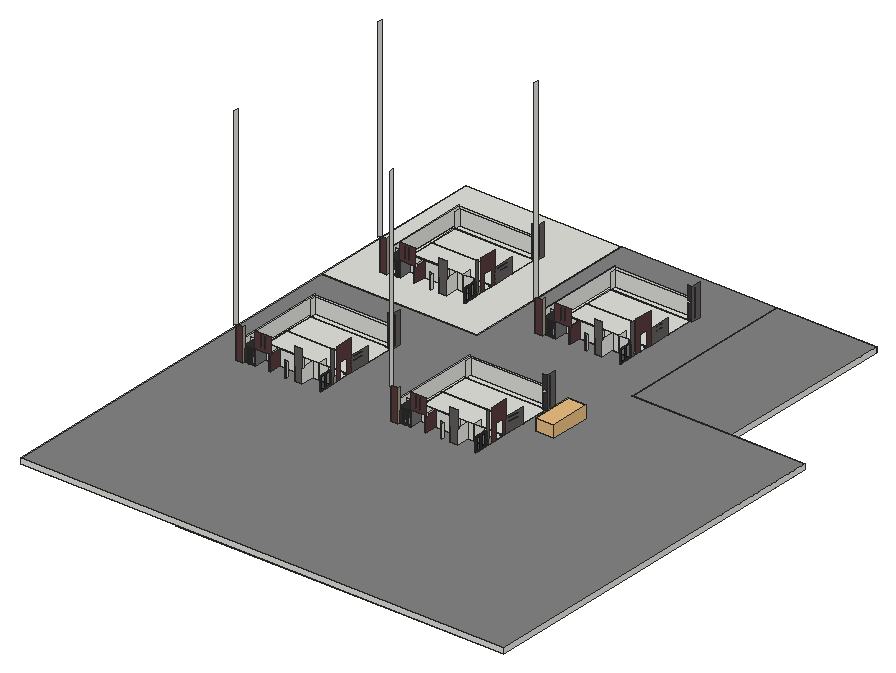
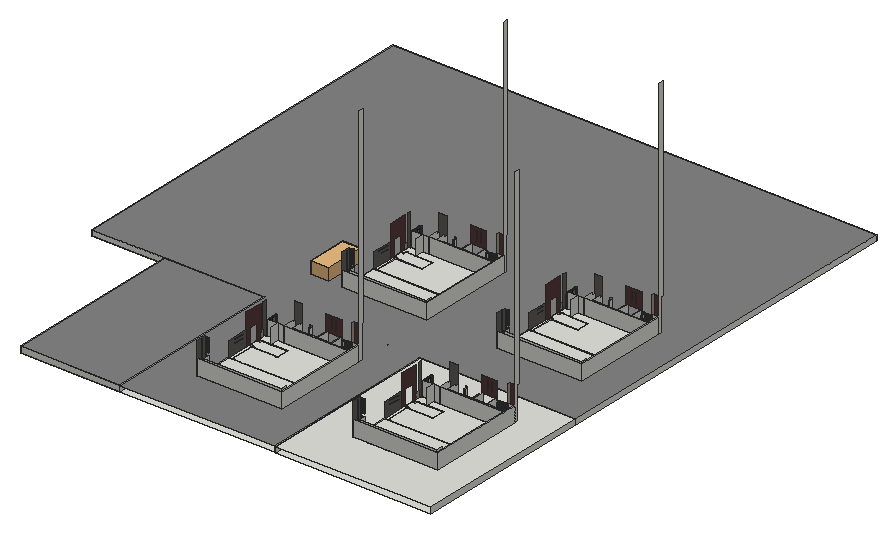
# SketchUp Ruby script. Lengths in inches.
U = 1.inch
M = Sketchup.active_model
def pt(a) = Geom::Point3d.new(a.map { |v| v * U })
def face(e, loops, mat)
  f = e.add_face(loops[0].map { |a| pt(a) })
  loops[1..].each { |l| e.add_face(l.map { |a| pt(a) }).erase! }
  f.material = f.back_material = mat if mat
  f
end
# faces: each face lists its corners as indices into pts; further lists are holes
def faces(e, pts, list, mat = nil) = list.each { |f| face(e, (f[0].is_a?(Array) ? f : [f]).map { |l| l.map { |i| pts[i] } }, mat) }
# xy, xz, yz: faces in a plane at the given z, y or x. An outline is a flat list of corners, or four numbers for a rectangle; further outlines are holes
def ring(l) = l.size == 4 ? [[l[0], l[1]], [l[2], l[1]], [l[2], l[3]], [l[0], l[3]]] : l.each_slice(2).to_a
def flat(e, list, mat, &to3) = list.each { |f| face(e, (f[0].is_a?(Array) ? f : [f]).map { |l| ring(l).map { |u, v| to3.(u, v) } }, mat) }
def xy(e, z, list, mat = nil) = flat(e, list, mat) { |x, y| [x, y, z] }
def xz(e, y, list, mat = nil) = flat(e, list, mat) { |x, z| [x, y, z] }
def yz(e, x, list, mat = nil) = flat(e, list, mat) { |y, z| [x, y, z] }
def lines(e, pts, list) = list.each { |a, b| e.add_line(pt(pts[a]), pt(pts[b])) }
# prism: a flat outline (further loops are holes) pulled along v
def prism(e, loops, v, mat = nil)
  f = face(e, loops, mat); d = Geom::Vector3d.new(v.map { |x| x * U })
  f.pushpull(f.normal.samedirection?(d) ? d.length : -d.length)
end
def box(e, o, s, mat = nil) = prism(e, [[o, [o[0] + s[0], o[1], o[2]], [o[0] + s[0], o[1] + s[1], o[2]], [o[0], o[1] + s[1], o[2]]]], [0, 0, s[2]], mat)
def at(x, y, z, deg = 0) = Geom::Transformation.translation(pt([x, y, z])) * Geom::Transformation.rotation(ORIGIN, Z_AXIS, deg.degrees)
def axes(o, x, y, z) = Geom::Transformation.new([*x, 0, *y, 0, *z, 0, *pt(o).to_a, 1])
def part(name) = M.definitions.add(name)
# library, detail: a bought-in or finely detailed component or shape, given as its bounding box
def library(name, o, s) = part(name).tap { |d| box(d.entities, o, s) }
def detail(e, o, s) = box(e.add_group.entities, o, s)
def put(e, d, t, mat = nil) = e.add_instance(d, t).tap { |i| i.material = mat if mat }
def group(e, t, mat = nil) = e.add_group.tap { |g| g.transformation = t; g.material = mat if mat }.entities
root = M.entities
M.materials.add("Glass_Tinted_Gray").color = [0, 0, 0]
M.materials["Glass_Tinted_Gray"].alpha = 0.125
M.materials.add("Wine2").color = [0, 0, 0]
M.materials["Wine2"].alpha = 0
M.materials.add("[0130_Gainsboro]").color = [39, 45, 50]
M.materials.add("[0135_DarkGray]").color = [81, 81, 81]
M.materials.add("[Color M05]").color = [114, 114, 114]
M.materials.add("[Color M07]").color = [58, 58, 58]
M.materials.add("[Concrete Tile]").color = [165, 155, 133]
M.materials.add("[Granite Brown]").color = [89, 59, 61]
M.materials.add("[Mirror 02]").color = [229, 229, 229]
M.materials.add("[Stone Marble]").color = [99, 95, 94]
M.materials.add("[Terrazzo Light Blue]").color = [196, 214, 227]
M.materials.add("[Tile Grey]").color = [132, 132, 132]
c1 = part("PENTEK_RP Fineline 50S_Sliding_DoorCase_E1")
box(c1.entities,[0,0,0],[1.51,3.66,99.27],"[0135_DarkGray]")
c2 = part("PENTEK_RP Fineline 50S_SlidingDooe_Case_E2")
box(c2.entities,[0,0,0],[96.25,3.66,1.51],"[0135_DarkGray]")
c3 = part("pentek_RP Fineline 50S_SlidingDoor_Case")
put(c3.entities,c1,at(97.76,0,0))
put(c3.entities,c2,at(1.51,0,0))
put(c3.entities,c1,at(0,0,0))
put(c3.entities,c2,at(1.51,0,97.76))
c4 = part("PENTEK_RP Fineline 50S_SlidingDoor_GlazingBead_2")
box(c4.entities,[0,0,0],[0.56,0.59,94.39],"[0135_DarkGray]")
c5 = part("PENTEK_RP Fineline 50S_SlidingDoor_Glass")
box(c5.entities,[0,0,0],[46.58,0.16,94.39],"Glass_Tinted_Gray")
c6 = part("PENTEK_RP Fineline 50S_SlidingDoor_GlazingBead")
box(c6.entities,[0,0,0],[45.47,0.59,0.56],"[0135_DarkGray]")
c7 = part("PENTEK_RP Fineline 50S_SlidingDoor_Leaf_E1")
xy(c7.entities,0,[[0,0,0.93,1.97],[0.93,1.57,1.49,1.97]],"[0135_DarkGray]")
xy(c7.entities,96.25,[[0,0,0.93,0,0.93,1.57,1.49,1.57,1.49,1.97,0,1.97]],"[0135_DarkGray]")
xz(c7.entities,0,[[0,0,0.93,96.25]],"[0135_DarkGray]")
xz(c7.entities,1.57,[[0.93,0,1.49,95.32],[0.93,95.32,1.49,96.25]],"[0135_DarkGray]")
xz(c7.entities,1.97,[[0,0,1.49,96.25]],"[0135_DarkGray]")
yz(c7.entities,0,[[0,0,1.97,96.25]],"[0135_DarkGray]")
yz(c7.entities,0.93,[[0,0,1.57,0.93],[0,0.93,1.57,95.32],[0,95.32,1.57,96.25]],"[0135_DarkGray]")
yz(c7.entities,1.49,[[1.57,0,1.97,95.32],[1.57,95.32,1.97,96.25]],"[0135_DarkGray]")
c8 = part("PENTEK_RP Fineline 50S_SlidingDoor_Leaf_E2")
xy(c8.entities,0,[[0,0,0,1.57,0.56,1.57,0.56,1.97,46.02,1.97,46.02,1.57,46.58,1.57,46.58,0]],"[0135_DarkGray]")
xy(c8.entities,0.93,[[0,0,46.58,1.57]],"[0135_DarkGray]")
xy(c8.entities,1.49,[[0.56,1.57,46.02,1.97]],"[0135_DarkGray]")
xz(c8.entities,0,[[0,0,46.58,0.93]],"[0135_DarkGray]")
xz(c8.entities,1.57,[[0,0,0.56,0.93],[46.02,0,46.58,0.93],[0.56,0.93,46.02,1.49]],"[0135_DarkGray]")
xz(c8.entities,1.97,[[0.56,0,46.02,1.49]],"[0135_DarkGray]")
yz(c8.entities,0,[[0,0,1.57,0.93]],"[0135_DarkGray]")
yz(c8.entities,0.56,[[1.57,0,1.97,0.93],[1.57,0.93,1.97,1.49]],"[0135_DarkGray]")
yz(c8.entities,46.02,[[1.57,0,1.97,0.93],[1.57,0.93,1.97,1.49]],"[0135_DarkGray]")
yz(c8.entities,46.58,[[0,0,1.57,0.93]],"[0135_DarkGray]")
c9 = part("PENTEK_RP Fineline S_SlidingDoor_Leaf1")
put(c9.entities,c4,at(0.93,0,0.93))
put(c9.entities,c4,at(46.96,0,0.93))
put(c9.entities,c5,at(1.49,1.42,0.93))
put(c9.entities,c6,at(1.49,0,0.93))
put(c9.entities,c5,at(1.49,0.59,0.93),"[Terrazzo Light Blue]")
put(c9.entities,c7,at(0,0,0))
put(c9.entities,c7,axes([48.44,0,0],[-1,0,0],[0,1,0],[0,0,1]))
put(c9.entities,c8,axes([0.93,0,96.25],[1,0,0],[0,1,0],[0,0,-1]))
put(c9.entities,c8,at(0.93,0,0))
put(c9.entities,c6,at(1.49,0,94.77))
c10 = part("PENTEK_RP Fineline 50S_SlidingDoor_Leaf2")
put(c10.entities,c5,at(1.49,1.42,0.93))
put(c10.entities,c6,at(1.49,0,94.77))
put(c10.entities,c4,at(46.96,0,0.93))
put(c10.entities,c5,at(1.49,0.59,0.93),"[Mirror 02]")
put(c10.entities,c4,at(0.93,0,0.93))
put(c10.entities,c7,at(0,0,0))
put(c10.entities,c7,axes([48.44,0,0],[-1,0,0],[0,1,0],[0,0,1]))
put(c10.entities,c6,at(1.49,0,0.93))
put(c10.entities,c8,axes([0.93,0,96.25],[1,0,0],[0,1,0],[0,0,-1]))
put(c10.entities,c8,at(0.93,0,0))
c11 = part("PENTEK - Slimmest Steel Sliding Door / Window\#1")
put(c11.entities,c3,at(0,-1.88,-0.09))
put(c11.entities,c9,at(1.51,-2.27,1.42))
put(c11.entities,c10,at(49.32,-0.3,1.42))
c12 = library("Group\#4",[0,0,0],[85.51,189.4,58.01])
c13 = part("2022 BMW i4")
put(c13.entities,c12,axes([0,0,0],[5,0,0],[0,5,0],[0,0,5]))
c14 = part("Framed glazing panel")
xy(c14.entities,0,[[0,-0.98,43.07,0],[0,0,43.07,1.4]],"[0130_Gainsboro]")
xy(c14.entities,0.3,[[0.3,-1.43,42.77,-0.98]],"[0130_Gainsboro]")
xy(c14.entities,2.95,[[2.95,-1.43,40.12,-0.63],[2.95,-0.63,40.12,0],[2.95,0,40.12,0.64],[2.95,0.64,40.12,1.4]],"[0130_Gainsboro]")
xy(c14.entities,3.54,[[3.54,-0.63,39.53,0],[3.54,0,39.53,0.64]],"[0130_Gainsboro]")
xy(c14.entities,111.8125,[[3.54,-0.63,39.53,0],[3.54,0,39.53,0.64]],"[0130_Gainsboro]")
xy(c14.entities,112.4,[[2.95,-1.43,40.12,-0.63],[2.95,-0.63,40.12,0],[2.95,0,40.12,0.64],[2.95,0.64,40.12,1.4]],"[0130_Gainsboro]")
xy(c14.entities,115.05,[[0.3,-1.43,42.77,-0.98]],"[0130_Gainsboro]")
xy(c14.entities,115.35,[[0,-0.98,43.07,0],[0,0,43.07,1.4]],"[0130_Gainsboro]")
xz(c14.entities,-1.43,[[[0.3,0.3,42.77,115.05],[2.95,2.95,40.12,112.4]]],"[0130_Gainsboro]")
xz(c14.entities,-0.98,[[[0,0,43.07,115.35],[0.3,0.3,42.77,115.05]]],"[0130_Gainsboro]")
xz(c14.entities,-0.63,[[[2.95,2.95,40.12,112.4],[3.54,3.54,39.53,111.8125]]],"[0130_Gainsboro]")
xz(c14.entities,0,[[3.54,3.54,39.53,111.8125]],"Wine2")
xz(c14.entities,0,[[[0,0,43.07,115.35],[2.95,2.95,40.12,112.4]],[[2.95,2.95,40.12,112.4],[3.54,3.54,39.53,111.8125]]],"[0130_Gainsboro]")
xz(c14.entities,0.64,[[[2.95,2.95,40.12,112.4],[3.54,3.54,39.53,111.8125]]],"[0130_Gainsboro]")
xz(c14.entities,1.4,[[[0,0,43.07,115.35],[2.95,2.95,40.12,112.4]]],"[0130_Gainsboro]")
yz(c14.entities,0,[[-0.98,0,0,115.35],[0,0,1.4,115.35]],"[0130_Gainsboro]")
yz(c14.entities,0.3,[[-1.43,0.3,-0.98,115.05]],"[0130_Gainsboro]")
yz(c14.entities,2.95,[[-1.43,2.95,-0.63,112.4],[-0.63,2.95,0,112.4],[0,2.95,0.64,112.4],[0.64,2.95,1.4,112.4]],"[0130_Gainsboro]")
yz(c14.entities,3.54,[[-0.63,3.54,0,111.8125],[0,3.54,0.64,111.8125]],"[0130_Gainsboro]")
yz(c14.entities,39.53,[[-0.63,3.54,0,111.8125],[0,3.54,0.64,111.8125]],"[0130_Gainsboro]")
yz(c14.entities,40.12,[[-1.43,2.95,-0.63,112.4],[-0.63,2.95,0,112.4],[0,2.95,0.64,112.4],[0.64,2.95,1.4,112.4]],"[0130_Gainsboro]")
yz(c14.entities,42.77,[[-1.43,0.3,-0.98,115.05]],"[0130_Gainsboro]")
yz(c14.entities,43.07,[[-0.98,0,0,115.35],[0,0,1.4,115.35]],"[0130_Gainsboro]")
c15 = part("Glazed panel assembly")
put(c15.entities,c14,axes([90.57,1.43,0],[1.05148,0,0],[0,1,0],[0,0,1]))
put(c15.entities,c14,axes([0,1.43,0],[1.05148,0,0],[0,1,0],[0,0,1]))
put(c15.entities,c14,axes([45.29,1.43,0],[1.05148,0,0],[0,1,0],[0,0,1]))
xy(root,-36.6875,[[0,0,1218.1875,2946.875],[1218.1875,0,1220.8125,2946.875],[1220.8125,0,3787.0625,2946.875],[0,2946.875,1218.1875,4361.5625],[1218.1875,2946.875,1220.8125,4361.5625],
  [1220.8125,2946.875,2436.375,4361.5625],[2439,2946.875,3218.5,4361.5625]])
xy(root,6,[[262.875,1778.3125,319.53,1799.9375],[1481.0625,1778.3125,1537.72,1799.9375],[262.875,1799.9375,262.875,2554.375,927.75,2554.375,927.75,2483.21,890.875,2483.21,890.875,2531.375,285.875,2531.375,285.875,1902.66,767.19,1902.66,767.19,1799.9375,709.87,1799.9375,709.87,1893.25,521.59,1893.25,521.59,1799.9375,511.23,1799.9375,511.23,1893.25,406.68,1893.25,406.68,1799.9375,399.88,1799.9375,399.88,1893.25,319.53,1893.25,319.53,1799.9375],[634.11,1799.9375,647.8,1814.92],[1481.0625,1799.9375,1481.0625,2554.375,2145.9375,2554.375,2145.9375,2483.21,2109.0625,2483.21,2109.0625,2531.375,1504.0625,2531.375,1504.0625,1902.66,1985.38,1902.66,1985.38,1799.9375,1928.05,1799.9375,1928.05,1893.25,1739.78,1893.25,1739.78,1799.9375,1729.42,1799.9375,1729.42,1893.25,1624.87,1893.25,1624.87,1799.9375,1618.07,1799.9375,1618.07,1893.25,1537.72,1893.25,1537.72,1799.9375],
  [1852.3,1799.9375,1865.99,1814.92],[285.875,1902.66,817,1902.66,817,1970.91,683.6875,1970.91,683.6875,2070.28,890.875,2070.28,890.875,2257.8125,285.875,2257.8125],[817,1902.66,817,1970.91,890.875,1970.91,890.875,1987.85,913.875,1987.85,913.875,1902.66],[1504.0625,1902.66,2035.1875,1902.66,2035.1875,1970.91,1901.875,1970.91,1901.875,2070.28,2109.0625,2070.28,2109.0625,2257.8125,1504.0625,2257.8125],[2035.1875,1902.66,2035.1875,1970.91,2109.0625,1970.91,2109.0625,1987.85,2132.0625,1987.85,2132.0625,1902.66],
  [683.6875,1970.91,683.6875,2070.28,890.875,2070.28,890.875,2059.15,913.875,2059.15,913.875,1987.85,890.875,1987.85,890.875,1970.91],[1901.875,1970.91,1901.875,2070.28,2109.0625,2070.28,2109.0625,2059.15,2132.0625,2059.15,2132.0625,1987.85,2109.0625,1987.85,2109.0625,1970.91],[890.875,2059.15,913.875,2257.8125],[2109.0625,2059.15,2132.0625,2257.8125],[285.875,2257.8125,285.875,2485.84,890.875,2485.84,890.875,2483.21,913.875,2483.21,913.875,2257.8125],
  [1504.0625,2257.8125,1504.0625,2485.84,2109.0625,2485.84,2109.0625,2483.21,2132.0625,2483.21,2132.0625,2257.8125],[285.875,2485.84,890.875,2531.375],[1504.0625,2485.84,2109.0625,2531.375],[0,2946.875,1218.1875,2946.875,1218.1875,4361.5625,262.875,4361.5625,262.875,3969.0625,927.75,3969.0625,927.75,3897.9,913.875,3897.9,913.875,3317.34,767.19,3317.34,767.19,3214.625,709.87,3214.625,709.87,3307.9375,634.11,3307.9375,634.11,3229.61,647.8,3229.61,647.8,3214.625,634.11,3214.625,634.11,3307.9375,521.59,3307.9375,521.59,3214.625,511.23,3214.625,511.23,3307.9375,406.68,3307.9375,406.68,3214.625,399.88,3214.625,399.88,3307.9375,319.53,3307.9375,319.53,3193,262.875,3193,262.875,4361.5625,0,4361.5625],[1218.1875,2946.875,1220.8125,4361.5625],
  [262.875,3193,319.53,3214.625],[1481.0625,3193,1537.72,3214.625],[262.875,3214.625,262.875,3969.0625,927.75,3969.0625,927.75,3897.9,890.875,3897.9,890.875,3946.0625,285.875,3946.0625,285.875,3317.34,767.19,3317.34,767.19,3214.625,709.87,3214.625,709.87,3307.9375,521.59,3307.9375,521.59,3214.625,511.23,3214.625,511.23,3307.9375,406.68,3307.9375,406.68,3214.625,399.88,3214.625,399.88,3307.9375,319.53,3307.9375,319.53,3214.625],[634.11,3214.625,647.8,3229.61],[1481.0625,3214.625,1481.0625,3969.0625,2145.9375,3969.0625,2145.9375,3897.9,2109.0625,3897.9,2109.0625,3946.0625,1504.0625,3946.0625,1504.0625,3317.34,1985.38,3317.34,1985.38,3214.625,1928.05,3214.625,1928.05,3307.9375,1739.78,3307.9375,1739.78,3214.625,1729.42,3214.625,1729.42,3307.9375,1624.87,3307.9375,1624.87,3214.625,1618.07,3214.625,1618.07,3307.9375,1537.72,3307.9375,1537.72,3214.625],
  [1852.3,3214.625,1865.99,3229.61],[285.875,3317.34,817,3317.34,817,3385.6,683.6875,3385.6,683.6875,3484.97,890.875,3484.97,890.875,3672.5,285.875,3672.5],[817,3317.34,817,3385.6,890.875,3385.6,890.875,3402.54,913.875,3402.54,913.875,3317.34],[1504.0625,3317.34,2035.1875,3317.34,2035.1875,3385.6,1901.875,3385.6,1901.875,3484.97,2109.0625,3484.97,2109.0625,3672.5,1504.0625,3672.5],[2035.1875,3317.34,2035.1875,3385.6,2109.0625,3385.6,2109.0625,3402.54,2132.0625,3402.54,2132.0625,3317.34],
  [683.6875,3385.6,683.6875,3484.97,890.875,3484.97,890.875,3473.84,913.875,3473.84,913.875,3402.54,890.875,3402.54,890.875,3385.6],[1901.875,3385.6,1901.875,3484.97,2109.0625,3484.97,2109.0625,3473.84,2132.0625,3473.84,2132.0625,3402.54,2109.0625,3402.54,2109.0625,3385.6],[890.875,3473.84,913.875,3672.5],[2109.0625,3473.84,2132.0625,3672.5],[285.875,3672.5,285.875,3900.52,890.875,3900.52,890.875,3897.9,913.875,3897.9,913.875,3672.5],
  [1504.0625,3672.5,1504.0625,3900.52,2109.0625,3900.52,2109.0625,3897.9,2132.0625,3897.9,2132.0625,3672.5],[285.875,3900.52,890.875,3946.0625],[1504.0625,3900.52,2109.0625,3946.0625]])
xy(root,6,[[0,0,3787.0625,0,3787.0625,2946.875,2436.375,2946.875,2436.375,4361.5625,1481.0625,4361.5625,1481.0625,3969.0625,2145.9375,3969.0625,2145.9375,3897.9,2132.0625,3897.9,2132.0625,3317.34,1985.38,3317.34,1985.38,3214.625,1928.05,3214.625,1928.05,3307.9375,1852.3,3307.9375,1852.3,3229.61,1865.99,3229.61,1865.99,3214.625,1852.3,3214.625,1852.3,3307.9375,1739.78,3307.9375,1739.78,3214.625,1729.42,3214.625,1729.42,3307.9375,1624.87,3307.9375,1624.87,3214.625,1618.07,3214.625,1618.07,3307.9375,1537.72,3307.9375,1537.72,3193,1481.0625,3193,1481.0625,4361.5625,1220.8125,4361.5625,1220.8125,2946.875,1481.0625,2946.875,1481.0625,2554.375,2145.9375,2554.375,2145.9375,2483.21,2132.0625,2483.21,2132.0625,1902.66,1985.38,1902.66,1985.38,1799.9375,1928.05,1799.9375,1928.05,1893.25,1852.3,1893.25,1852.3,1814.92,1865.99,1814.92,1865.99,1799.9375,1852.3,1799.9375,1852.3,1893.25,1739.78,1893.25,1739.78,1799.9375,1729.42,1799.9375,1729.42,1893.25,1624.87,1893.25,1624.87,1799.9375,1618.07,1799.9375,1618.07,1893.25,1537.72,1893.25,1537.72,1778.3125,1481.0625,1778.3125,1481.0625,2946.875,262.875,2946.875,262.875,2554.375,927.75,2554.375,927.75,2483.21,913.875,2483.21,913.875,1902.66,767.19,1902.66,767.19,1799.9375,709.87,1799.9375,709.87,1893.25,634.11,1893.25,634.11,1814.92,647.8,1814.92,647.8,1799.9375,634.11,1799.9375,634.11,1893.25,521.59,1893.25,521.59,1799.9375,511.23,1799.9375,511.23,1893.25,406.68,1893.25,406.68,1799.9375,399.88,1799.9375,399.88,1893.25,319.53,1893.25,319.53,1778.3125,262.875,1778.3125,262.875,2946.875,0,2946.875],[2439,2946.875,3218.5,4361.5625]],"[Tile Grey]")
xz(root,0,[[0,-36.6875,3787.0625,6]])
xz(root,1778.3125,[[262.875,6,319.53,258],[1481.0625,6,1537.72,258]],"[Granite Brown]")
xz(root,1799.9375,[[262.875,6,319.53,126],[1481.0625,6,1537.72,126]])
xz(root,1799.9375,[[634.11,6,647.8,126],[1852.3,6,1865.99,126]],"[Concrete Tile]")
xz(root,1799.9375,[[399.88,6,406.68,126],[[511.23,6,521.59,6,521.59,252,399.88,252,399.88,126,511.23,126],[434.43,145.8125,450.49,240.875],[467.98,147.29,483.79,240.11]],[1618.07,6,1624.87,126],[[1729.42,6,1739.78,6,1739.78,252,1618.07,252,1618.07,126,1729.42,126],[1652.62,145.8125,1668.68,240.875],[1686.17,147.29,1701.98,240.11]]],"[Granite Brown]")
xz(root,1799.9375,[[709.87,6,767.19,252],[1928.05,6,1985.38,252]],"[Stone Marble]")
xz(root,1814.92,[[634.11,6,647.8,112.625],[1852.3,6,1865.99,112.625]])
xz(root,1893.25,[[319.53,6,399.88,126],[406.68,6,511.23,126],[521.59,6,634.11,126],[634.11,6,709.87,126],[1537.72,6,1618.07,126],
  [1624.87,6,1729.42,126],[1739.78,6,1852.3,126],[1852.3,6,1928.05,126]])
xz(root,1902.66,[[285.875,6,767.19,126],[767.19,6,817,126],[817,6,913.875,6,913.875,112.625,890.875,112.625,890.875,126,817,126],[1504.0625,6,1985.38,126],[1985.38,6,2035.1875,126],
  [2035.1875,6,2132.0625,6,2132.0625,112.625,2109.0625,112.625,2109.0625,126,2035.1875,126]])
xz(root,1970.91,[[683.6875,6,817,7.75],[817,6,890.875,7.75],[1901.875,6,2035.1875,7.75],[2035.1875,6,2109.0625,7.75]])
xz(root,1987.85,[[890.875,6,913.875,7.75],[2109.0625,6,2132.0625,7.75]])
xz(root,2059.15,[[890.875,6,913.875,7.75],[2109.0625,6,2132.0625,7.75]])
xz(root,2070.28,[[683.6875,6,890.875,7.75],[1901.875,6,2109.0625,7.75]])
xz(root,2257.8125,[[285.875,6,890.875,7.75],[890.875,6,913.875,7.75],[1504.0625,6,2109.0625,7.75],[2109.0625,6,2132.0625,7.75]])
xz(root,2483.21,[[890.875,6,913.875,7.75],[2109.0625,6,2132.0625,7.75]])
xz(root,2483.21,[[913.875,6,927.75,6,927.75,252,890.875,252,890.875,143.875,913.875,143.875,913.875,145.375,921.125,145.375,921.125,112.625,913.875,112.625,913.875,126,890.875,126,890.875,7.75,913.875,7.75],[2132.0625,6,2145.9375,6,2145.9375,252,2109.0625,252,2109.0625,143.875,2132.0625,143.875,2132.0625,145.375,2139.3125,145.375,2139.3125,112.625,2132.0625,112.625,2132.0625,126,2109.0625,126,2109.0625,7.75,2132.0625,7.75]],"[Color M07]")
xz(root,2485.84,[[285.875,6,890.875,7.75],[1504.0625,6,2109.0625,7.75]])
xz(root,2531.375,[[285.875,6,890.875,126],[1504.0625,6,2109.0625,126]])
xz(root,2554.375,[[262.875,6,262.875,126,913.875,126,913.875,120.4375,927.75,120.4375,927.75,6],[1481.0625,6,1481.0625,126,2132.0625,126,2132.0625,120.4375,2145.9375,120.4375,2145.9375,6]])
xz(root,2946.875,[[0,-36.6875,2.625,6],[2.625,-36.6875,1218.1875,6],[1218.1875,-36.6875,1220.8125,6],[2436.375,-36.6875,2439,6],[2439,-36.6875,3218.5,6],
  [3218.5,-36.6875,3787.0625,6]])
xz(root,3193,[[262.875,6,319.53,258],[1481.0625,6,1537.72,258]],"[Granite Brown]")
xz(root,3214.625,[[262.875,6,319.53,126],[1481.0625,6,1537.72,126]])
xz(root,3214.625,[[634.11,6,647.8,126],[1852.3,6,1865.99,126]],"[Concrete Tile]")
xz(root,3214.625,[[399.88,6,406.68,126],[[511.23,6,521.59,6,521.59,252,399.88,252,399.88,126,511.23,126],[434.43,145.8125,450.49,240.875],[467.98,147.29,483.79,240.11]],[1618.07,6,1624.87,126],[[1729.42,6,1739.78,6,1739.78,252,1618.07,252,1618.07,126,1729.42,126],[1652.62,145.8125,1668.68,240.875],[1686.17,147.29,1701.98,240.11]]],"[Granite Brown]")
xz(root,3214.625,[[709.87,6,767.19,252],[1928.05,6,1985.38,252]],"[Stone Marble]")
xz(root,3229.61,[[634.11,6,647.8,112.625],[1852.3,6,1865.99,112.625]])
xz(root,3307.9375,[[319.53,6,399.88,126],[406.68,6,511.23,126],[521.59,6,634.11,126],[634.11,6,709.87,126],[1537.72,6,1618.07,126],
  [1624.87,6,1729.42,126],[1739.78,6,1852.3,126],[1852.3,6,1928.05,126]])
xz(root,3317.34,[[285.875,6,767.19,126],[767.19,6,817,126],[817,6,913.875,6,913.875,112.625,890.875,112.625,890.875,126,817,126],[1504.0625,6,1985.38,126],[1985.38,6,2035.1875,126],
  [2035.1875,6,2132.0625,6,2132.0625,112.625,2109.0625,112.625,2109.0625,126,2035.1875,126]])
xz(root,3385.6,[[683.6875,6,817,7.75],[817,6,890.875,7.75],[1901.875,6,2035.1875,7.75],[2035.1875,6,2109.0625,7.75]])
xz(root,3402.54,[[890.875,6,913.875,7.75],[2109.0625,6,2132.0625,7.75]])
xz(root,3473.84,[[890.875,6,913.875,7.75],[2109.0625,6,2132.0625,7.75]])
xz(root,3484.97,[[683.6875,6,890.875,7.75],[1901.875,6,2109.0625,7.75]])
xz(root,3672.5,[[285.875,6,890.875,7.75],[890.875,6,913.875,7.75],[1504.0625,6,2109.0625,7.75],[2109.0625,6,2132.0625,7.75]])
xz(root,3897.9,[[890.875,6,913.875,7.75],[2109.0625,6,2132.0625,7.75]])
xz(root,3897.9,[[913.875,6,927.75,6,927.75,252,890.875,252,890.875,143.875,913.875,143.875,913.875,145.375,921.125,145.375,921.125,112.625,913.875,112.625,913.875,126,890.875,126,890.875,7.75,913.875,7.75],[2132.0625,6,2145.9375,6,2145.9375,252,2109.0625,252,2109.0625,143.875,2132.0625,143.875,2132.0625,145.375,2139.3125,145.375,2139.3125,112.625,2132.0625,112.625,2132.0625,126,2109.0625,126,2109.0625,7.75,2132.0625,7.75]],"[Color M07]")
xz(root,3900.52,[[285.875,6,890.875,7.75],[1504.0625,6,2109.0625,7.75]])
xz(root,3946.0625,[[285.875,6,890.875,126],[1504.0625,6,2109.0625,126]])
xz(root,3969.0625,[[262.875,6,262.875,126,913.875,126,913.875,120.4375,927.75,120.4375,927.75,6],[1481.0625,6,1481.0625,126,2132.0625,126,2132.0625,120.4375,2145.9375,120.4375,2145.9375,6]])
xz(root,4361.5625,[[1218.1875,-36.6875,1220.8125,6],[2436.375,-36.6875,3218.5,6]])
yz(root,0,[[0,-36.6875,2946.875,6],[2946.875,-36.6875,4361.5625,6]])
yz(root,262.875,[[1778.3125,6,1778.3125,258,1763.25,258,1763.25,1764,1799.9375,1764,1799.9375,132,2554.375,132,2554.375,126,1799.9375,126,1799.9375,6],[1799.9375,6,2554.375,126],[3193,6,3193,258,3177.9375,258,3177.9375,1764,3214.625,1764,3214.625,132,3969.0625,132,3969.0625,126,3214.625,126,3214.625,6],[3214.625,6,3969.0625,126]])
yz(root,285.875,[[1902.66,6,2257.8125,7.75],[2257.8125,6,2485.84,7.75],[2485.84,6,2531.375,126],[3317.34,6,3672.5,7.75],[3672.5,6,3900.52,7.75],
  [3900.52,6,3946.0625,126]])
yz(root,319.53,[[1799.9375,6,1893.25,6,1893.25,126,1811.4375,126,1811.4375,112.625,1799.9375,112.625],[3214.625,6,3307.9375,6,3307.9375,126,3226.125,126,3226.125,112.625,3214.625,112.625]],"[Color M07]")
yz(root,319.53,[[1778.3125,6,1799.9375,258],[3193,6,3214.625,258]],"[Concrete Tile]")
yz(root,399.88,[[1799.9375,6,1799.9375,112.625,1811.4375,112.625,1811.4375,126,1893.25,126,1893.25,6],[3214.625,6,3214.625,112.625,3226.125,112.625,3226.125,126,3307.9375,126,3307.9375,6]])
yz(root,406.68,[[1799.9375,6,1893.25,126],[3214.625,6,3307.9375,126]],"[Color M05]")
yz(root,511.23,[[1799.9375,6,1893.25,126],[3214.625,6,3307.9375,126]])
yz(root,521.59,[[1799.9375,6,1893.25,6,1893.25,126,1822.9375,126,1822.9375,112.625,1799.9375,112.625],[3214.625,6,3307.9375,6,3307.9375,126,3237.625,126,3237.625,112.625,3214.625,112.625]],"[Granite Brown]")
yz(root,634.11,[[1799.9375,6,1814.92,112.625],[3214.625,6,3229.61,112.625]])
yz(root,647.8,[[1799.9375,6,1814.92,112.625],[3214.625,6,3229.61,112.625]])
yz(root,683.6875,[[1970.91,6,2070.28,7.75],[3385.6,6,3484.97,7.75]])
yz(root,709.87,[[1799.9375,6,1799.9375,112.625,1822.9375,112.625,1822.9375,126,1893.25,126,1893.25,6],[3214.625,6,3214.625,112.625,3237.625,112.625,3237.625,126,3307.9375,126,3307.9375,6]])
yz(root,767.19,[[1799.9375,6,1902.66,6,1902.66,126,1822.9375,126,1822.9375,112.625,1799.9375,112.625],[3214.625,6,3317.34,6,3317.34,126,3237.625,126,3237.625,112.625,3214.625,112.625]])
yz(root,817,[[1902.66,6,1970.91,126],[3317.34,6,3385.6,126]])
yz(root,890.875,[[1970.91,6,1987.85,7.75],[2059.15,6,2070.28,7.75],[2070.28,6,2257.8125,7.75],[2483.21,6,2485.84,7.75],[[2485.84,6,2531.375,126],[2497.47,13.21,2514.84,112.625]],
  [3385.6,6,3402.54,7.75],[3473.84,6,3484.97,7.75],[3484.97,6,3672.5,7.75],[3897.9,6,3900.52,7.75],[[3900.52,6,3946.0625,126],[3912.16,13.21,3929.52,112.625]]])
yz(root,913.875,[[1987.85,6,2059.15,7.75],[2257.8125,6,2483.21,7.75],[3402.54,6,3473.84,7.75],[3672.5,6,3897.9,7.75]])
yz(root,913.875,[[1926.07,6,1953.7,54.8],[3340.76,6,3368.39,54.8]],"[Concrete Tile]")
yz(root,913.875,[[1953.7,6,1987.85,6,1987.85,126,2059.15,126,2059.15,6,2093.65,6,2093.65,252,1953.7,252],[3368.39,6,3402.54,6,3402.54,126,3473.84,126,3473.84,6,3508.34,6,3508.34,252,3368.39,252]],"[Granite Brown]")
yz(root,913.875,[[1902.66,6,1926.07,252],[[2093.65,6,2257.8125,126],[2113.57,103.85,2213.62,117.41],[2113.57,76.14,2213.62,88.32]],[3317.34,6,3340.76,252],[[3508.34,6,3672.5,126],[3528.25,103.85,3628.31,117.41],[3528.25,76.14,3628.31,88.32]]],"[Stone Marble]")
yz(root,927.75,[[[2483.21,6,2554.375,252],[2497.47,13.21,2514.84,245.15]],[[3897.9,6,3969.0625,252],[3912.16,13.21,3929.52,245.15]]],"[Stone Marble]")
yz(root,1218.1875,[[2946.875,-36.6875,4361.5625,6]])
yz(root,1220.8125,[[2946.875,-36.6875,4361.5625,6]])
yz(root,1481.0625,[[1778.3125,6,1778.3125,258,1763.25,258,1763.25,1764,1799.9375,1764,1799.9375,132,2554.375,132,2554.375,126,1799.9375,126,1799.9375,6],[1799.9375,6,2554.375,126],[3193,6,3193,258,3177.9375,258,3177.9375,1764,3214.625,1764,3214.625,132,3969.0625,132,3969.0625,126,3214.625,126,3214.625,6],[3214.625,6,3969.0625,126]])
yz(root,1504.0625,[[1902.66,6,2257.8125,7.75],[2257.8125,6,2485.84,7.75],[2485.84,6,2531.375,126],[3317.34,6,3672.5,7.75],[3672.5,6,3900.52,7.75],
  [3900.52,6,3946.0625,126]])
yz(root,1537.72,[[1799.9375,6,1893.25,6,1893.25,126,1811.4375,126,1811.4375,112.625,1799.9375,112.625],[3214.625,6,3307.9375,6,3307.9375,126,3226.125,126,3226.125,112.625,3214.625,112.625]],"[Color M07]")
yz(root,1537.72,[[1778.3125,6,1799.9375,258],[3193,6,3214.625,258]],"[Concrete Tile]")
yz(root,1618.07,[[1799.9375,6,1799.9375,112.625,1811.4375,112.625,1811.4375,126,1893.25,126,1893.25,6],[3214.625,6,3214.625,112.625,3226.125,112.625,3226.125,126,3307.9375,126,3307.9375,6]])
yz(root,1624.87,[[1799.9375,6,1893.25,126],[3214.625,6,3307.9375,126]],"[Color M05]")
yz(root,1729.42,[[1799.9375,6,1893.25,126],[3214.625,6,3307.9375,126]])
yz(root,1739.78,[[1799.9375,6,1893.25,6,1893.25,126,1822.9375,126,1822.9375,112.625,1799.9375,112.625],[3214.625,6,3307.9375,6,3307.9375,126,3237.625,126,3237.625,112.625,3214.625,112.625]],"[Granite Brown]")
yz(root,1852.3,[[1799.9375,6,1814.92,112.625],[3214.625,6,3229.61,112.625]])
yz(root,1865.99,[[1799.9375,6,1814.92,112.625],[3214.625,6,3229.61,112.625]])
yz(root,1901.875,[[1970.91,6,2070.28,7.75],[3385.6,6,3484.97,7.75]])
yz(root,1928.05,[[1799.9375,6,1799.9375,112.625,1822.9375,112.625,1822.9375,126,1893.25,126,1893.25,6],[3214.625,6,3214.625,112.625,3237.625,112.625,3237.625,126,3307.9375,126,3307.9375,6]])
yz(root,1985.38,[[1799.9375,6,1902.66,6,1902.66,126,1822.9375,126,1822.9375,112.625,1799.9375,112.625],[3214.625,6,3317.34,6,3317.34,126,3237.625,126,3237.625,112.625,3214.625,112.625]])
yz(root,2035.1875,[[1902.66,6,1970.91,126],[3317.34,6,3385.6,126]])
yz(root,2109.0625,[[1970.91,6,1987.85,7.75],[2059.15,6,2070.28,7.75],[2070.28,6,2257.8125,7.75],[2483.21,6,2485.84,7.75],[[2485.84,6,2531.375,126],[2497.47,13.21,2514.84,112.625]],
  [3385.6,6,3402.54,7.75],[3473.84,6,3484.97,7.75],[3484.97,6,3672.5,7.75],[3897.9,6,3900.52,7.75],[[3900.52,6,3946.0625,126],[3912.16,13.21,3929.52,112.625]]])
yz(root,2132.0625,[[1987.85,6,2059.15,7.75],[2257.8125,6,2483.21,7.75],[3402.54,6,3473.84,7.75],[3672.5,6,3897.9,7.75]])
yz(root,2132.0625,[[1926.07,6,1953.7,54.8],[3340.76,6,3368.39,54.8]],"[Concrete Tile]")
yz(root,2132.0625,[[1953.7,6,1987.85,6,1987.85,126,2059.15,126,2059.15,6,2093.65,6,2093.65,252,1953.7,252],[3368.39,6,3402.54,6,3402.54,126,3473.84,126,3473.84,6,3508.34,6,3508.34,252,3368.39,252]],"[Granite Brown]")
yz(root,2132.0625,[[1902.66,6,1926.07,252],[[2093.65,6,2257.8125,126],[2113.57,103.85,2213.62,117.41],[2113.57,76.14,2213.62,88.32]],[3317.34,6,3340.76,252],[[3508.34,6,3672.5,126],[3528.25,103.85,3628.31,117.41],[3528.25,76.14,3628.31,88.32]]],"[Stone Marble]")
yz(root,2145.9375,[[[2483.21,6,2554.375,252],[2497.47,13.21,2514.84,245.15]],[[3897.9,6,3969.0625,252],[3912.16,13.21,3929.52,245.15]]],"[Stone Marble]")
yz(root,2439,[[2946.875,-36.6875,4361.5625,6]])
yz(root,3218.5,[[2946.875,-36.6875,4361.5625,6]])
yz(root,3787.0625,[[0,-36.6875,2946.875,6]])
p = [[-12383.22,-15329.6,-1273.76],[-12383.22,22406.65,-1273.76],[36035.72,22406.65,-1273.76],[36035.72,-15329.6,-1273.76]]
lines(root,p,[[0,1],[1,2],[2,3],[3,0]])
put(root,c11,axes([2127.76,1799.9375,4.5],[0,1.02084,0],[-2.51374,0,0],[0,0,1.05725]))
put(root,c11,axes([909.57,1799.9375,4.5],[0,1.02084,0],[-2.51374,0,0],[0,0,1.05725]))
put(root,c11,axes([2127.76,3214.625,4.5],[0,1.02084,0],[-2.51374,0,0],[0,0,1.05725]))
put(root,c11,axes([909.57,3214.625,4.5],[0,1.02084,0],[-2.51374,0,0],[0,0,1.05725]))
put(root,c13,axes([2253.11,2237.31,6],[0.33,0,0],[0,0.33,0],[0,0,0.33]))
put(root,c15,axes([1534.33,1799.9375,7.03],[0.61638,0,0],[0,1,0],[0,0,0.91782]))
put(root,c15,axes([316.14,1799.9375,7.03],[0.61638,0,0],[0,1,0],[0,0,0.91782]))
put(root,c15,axes([1534.33,3214.625,7.03],[0.61638,0,0],[0,1,0],[0,0,0.91782]))
put(root,c15,axes([316.14,3214.625,7.03],[0.61638,0,0],[0,1,0],[0,0,0.91782]))
